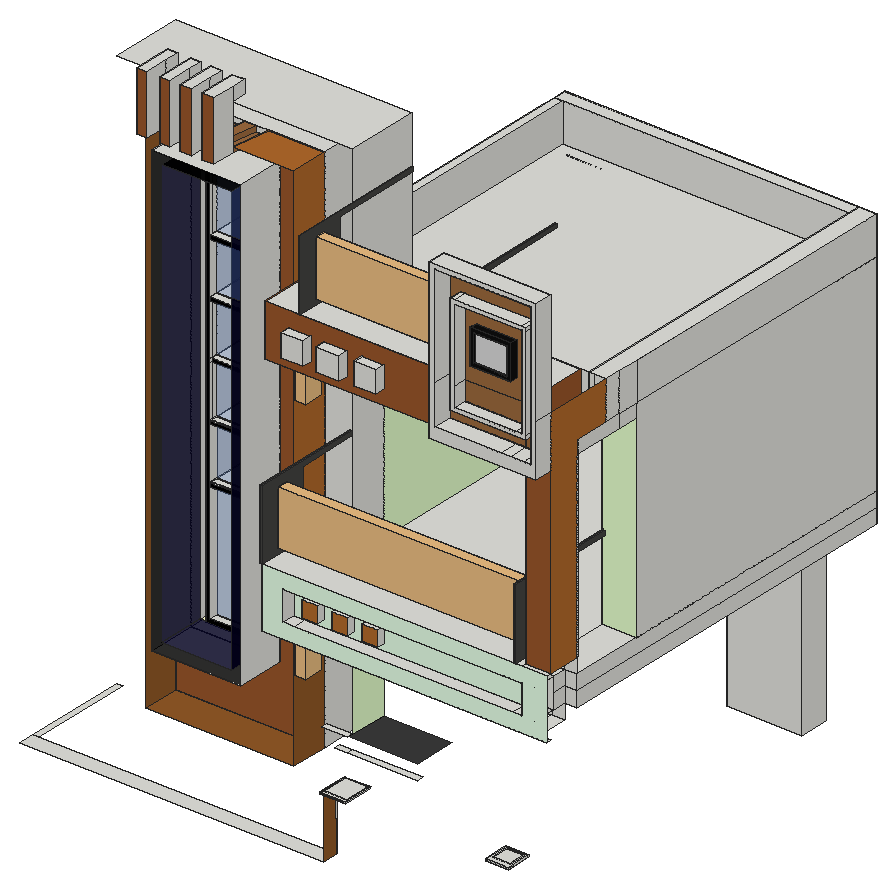
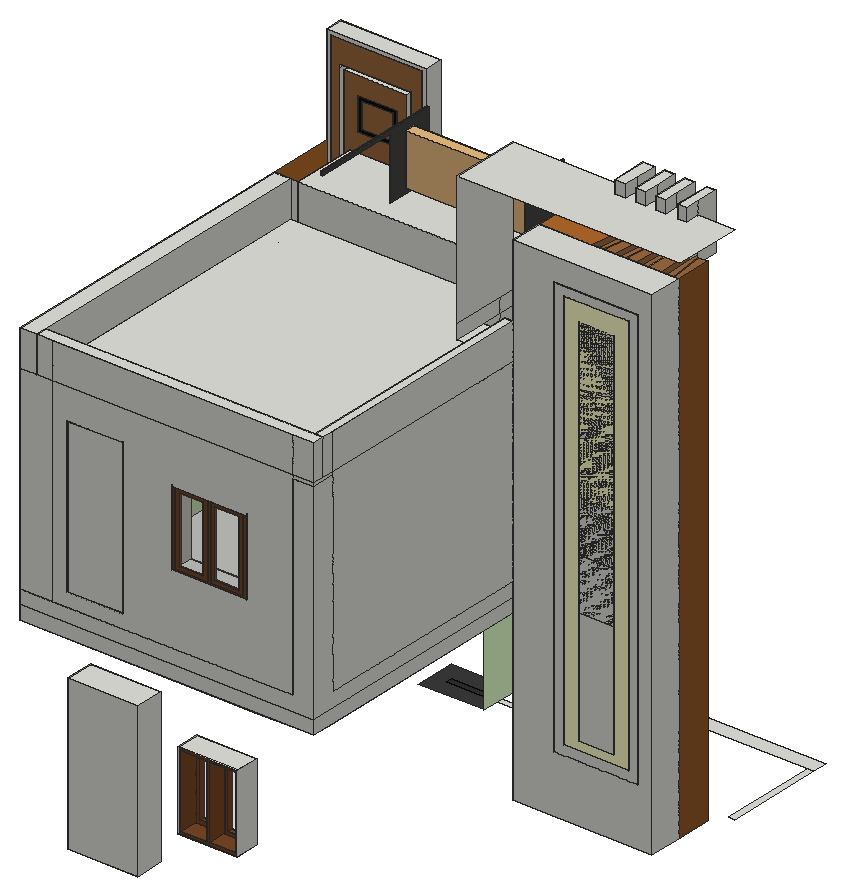
# SketchUp Ruby script. Lengths in inches.
U = 1.inch
M = Sketchup.active_model
def pt(a) = Geom::Point3d.new(a.map { |v| v * U })
def face(e, loops, mat)
  f = e.add_face(loops[0].map { |a| pt(a) })
  loops[1..].each { |l| e.add_face(l.map { |a| pt(a) }).erase! }
  f.material = f.back_material = mat if mat
  f
end
# faces: each face lists its corners as indices into pts; further lists are holes
def faces(e, pts, list, mat = nil) = list.each { |f| face(e, (f[0].is_a?(Array) ? f : [f]).map { |l| l.map { |i| pts[i] } }, mat) }
# xy, xz, yz: faces in a plane at the given z, y or x. An outline is a flat list of corners, or four numbers for a rectangle; further outlines are holes
def ring(l) = l.size == 4 ? [[l[0], l[1]], [l[2], l[1]], [l[2], l[3]], [l[0], l[3]]] : l.each_slice(2).to_a
def flat(e, list, mat, &to3) = list.each { |f| face(e, (f[0].is_a?(Array) ? f : [f]).map { |l| ring(l).map { |u, v| to3.(u, v) } }, mat) }
def xy(e, z, list, mat = nil) = flat(e, list, mat) { |x, y| [x, y, z] }
def xz(e, y, list, mat = nil) = flat(e, list, mat) { |x, z| [x, y, z] }
def yz(e, x, list, mat = nil) = flat(e, list, mat) { |y, z| [x, y, z] }
def lines(e, pts, list) = list.each { |a, b| e.add_line(pt(pts[a]), pt(pts[b])) }
# prism: a flat outline (further loops are holes) pulled along v
def prism(e, loops, v, mat = nil)
  f = face(e, loops, mat); d = Geom::Vector3d.new(v.map { |x| x * U })
  f.pushpull(f.normal.samedirection?(d) ? d.length : -d.length)
end
def box(e, o, s, mat = nil) = prism(e, [[o, [o[0] + s[0], o[1], o[2]], [o[0] + s[0], o[1] + s[1], o[2]], [o[0], o[1] + s[1], o[2]]]], [0, 0, s[2]], mat)
def at(x, y, z, deg = 0) = Geom::Transformation.translation(pt([x, y, z])) * Geom::Transformation.rotation(ORIGIN, Z_AXIS, deg.degrees)
def axes(o, x, y, z) = Geom::Transformation.new([*x, 0, *y, 0, *z, 0, *pt(o).to_a, 1])
def part(name) = M.definitions.add(name)
# library, detail: a bought-in or finely detailed component or shape, given as its bounding box
def library(name, o, s) = part(name).tap { |d| box(d.entities, o, s) }
def detail(e, o, s) = box(e.add_group.entities, o, s)
def put(e, d, t, mat = nil) = e.add_instance(d, t).tap { |i| i.material = mat if mat }
def group(e, t, mat = nil) = e.add_group.tap { |g| g.transformation = t; g.material = mat if mat }.entities
root = M.entities
M.materials.add("MOLDURA PRETA").color = [15, 15, 15]
M.materials.add("[Color E01]").color = [255, 255, 204]
M.materials.add("[Color E03]").color = [229, 255, 230]
M.materials.add("[Color F01]1").color = [229, 255, 204]
M.materials.add("[Color I07]").color = [0, 0, 0]
M.materials["[Color I07]"].alpha = 0.79
M.materials.add("[Color J08]").color = [2, 0, 36]
M.materials["[Color J08]"].alpha = 0.79
M.materials.add("[Color M09]").color = [0, 0, 0]
M.materials.add("[Metal Seamed]2").color = [68, 68, 66]
M.materials.add("[Translucent Glass Blue]").color = [100, 149, 237]
M.materials["[Translucent Glass Blue]"].alpha = 0.28
M.materials.add("[Translucent Glass Gray]").color = [132, 132, 132]
M.materials["[Translucent Glass Gray]"].alpha = 0.25
M.materials.add("[Wood Bamboo]").color = [177, 105, 43]
M.materials.add("[Wood Cherry Original]").color = [152, 86, 42]
M.materials.add("[Wood Floor Parquet]").color = [145, 89, 39]
M.materials.add("[Wood Floor]").color = [155, 105, 61]
M.materials.add("[Wood Veneer 01]").color = [120, 70, 37]
M.materials.add("arvore preta").color = [217, 217, 217]
c1 = part("DOOR12")
g1 = group(c1.entities,at(114.73,28.14,-0.51))
g2 = group(g1,at(0,0,0))
box(g2,[0,0,0],[36,0.5,77.7])
c2 = part("Group\#8")
xy(c2.entities,0,[[0,0,19.69,1.18]],"[Wood Veneer 01]")
xy(c2.entities,2.76,[[2.76,0,16.93,1.18]],"[Wood Veneer 01]")
xy(c2.entities,60.24,[[2.76,0,16.93,1.18]],"[Wood Veneer 01]")
xy(c2.entities,62.99,[[0,0,19.69,1.18]],"[Wood Veneer 01]")
xz(c2.entities,0,[[2.76,2.76,16.93,60.24]],"[Translucent Glass Gray]")
xz(c2.entities,0,[[[0,0,19.69,62.99],[2.76,2.76,16.93,60.24]]],"[Wood Veneer 01]")
xz(c2.entities,1.18,[[[0,0,19.69,62.99],[2.76,2.76,16.93,60.24]]],"[Wood Veneer 01]")
yz(c2.entities,0,[[0,0,1.18,62.99]],"[Wood Veneer 01]")
yz(c2.entities,2.76,[[0,2.76,1.18,60.24]],"[Wood Veneer 01]")
yz(c2.entities,16.93,[[0,2.76,1.18,60.24]],"[Wood Veneer 01]")
yz(c2.entities,19.69,[[0,0,1.18,62.99]],"[Wood Veneer 01]")
c3 = part("pintu 2")
put(c3.entities,c2,at(-19.69,0,1.97))
g3 = group(c3.entities,at(-21.65,0,0))
prism(g3,[[[0,0,66.93],[0,0,0],[45.28,0,0],[45.28,0,66.93]],[[43.31,0,1.97],[23.62,0,1.97],[23.62,0,64.96],[43.31,0,64.96]],[[21.65,0,64.96],[21.65,0,1.97],[1.97,0,1.97],[1.97,0,64.96]]],[0,5.91,0],"[Wood Veneer 01]")
put(c3.entities,c2,at(1.97,0,1.97))
c4 = library("Wall+Light",[81.37,10.74,0],[4.72,6.69,7.875])
c5 = part("Vertical support bracket")
prism(c5.entities,[[[0.39,10.04,41.34],[0.39,0,41.34],[0.39,0,0],[0.39,3.54,0],[0.39,3.54,38.58],[0.39,10.04,38.98]]],[-0.39,0,0],"[Metal Seamed]2")
c6 = part("Link_to_node_rj4\#1")
put(c6.entities,c5,at(2.36,0,0))
c7 = part("Link_to_node_rj8\#1")
put(c7.entities,c5,at(-2.36,0,0),"[Metal Seamed]2")
c8 = library("Horizontal grille bars",[-150.39,-2.17,3.54],[41.02,0.79,32.29])
c9 = part("Agrupar\#1")
prism(c9.entities,[[[14.17,0,12.2],[0,0,12.2],[0,0,0],[14.17,0,0]],[[1.18,0,1.18],[1.18,0,11.02],[12.99,0,11.02],[12.99,0,1.18]]],[0,0.79,0])
c10 = part("Agrupar\#4")
xz(c10.entities,0,[[0,0,11.8125,9.84]],"arvore preta")
c11 = part("Agrupar\#6")
put(c11.entities,c9,at(0,0,0),"MOLDURA PRETA")
put(c11.entities,c10,at(1.18,0.2,1.18))
xy(root,12.68,[[11.58,65.625,71,79.8125]])
xy(root,12.68,[[11.58,50.4375,71,65.625]],"[Wood Floor Parquet]")
xy(root,17.375,[[0,2.125,121.48,8.54],[0,8.54,2.44,50.4375]])
xy(root,26.05,[[103.63,175.125,128.94,185.625]])
xy(root,26.81,[[89.3,47.875,94.55,50.4375],[94.55,47.875,122.48,50.4375]])
xy(root,32.52,[[84.05,47.875,94.55,50.4375]])
xy(root,32.52,[[94.55,47.875,122.48,65.625]],"[Color I07]")
xy(root,37.35,[[17.51,46.0625,53.28,65.625],[17.51,65.625,53.28,79.8125]])
xy(root,41.3,[[21.46,65.625,49.33,79.8125]],"[Color E01]")
xy(root,41.3,[[21.46,46.0625,49.33,65.625]],"[Color J08]")
xy(root,42.0625,[[[187.91,0,197.0625,10.15],[189.03,2.125,196.0625,9.15]]])
xy(root,42.1875,[[120.98,0.77,131.48,2.125],[120.99,2.125,121.48,12.5],[130.61,2.125,131.48,12.75]])
xy(root,42.8125,[[[187.91,0,197.0625,10.15],[189.03,2.125,196.0625,9.15]],[120.98,0.77,131.48,2.125],[120.99,2.125,121.48,12.5],[121.48,2.125,130.61,2.125,130.61,12.75,121.49,12.5,121.49,8.29,121.48,8.54],[130.61,2.125,131.48,12.75],
  [189.03,2.125,196.0625,9.15],[121.49,8.29,121.49,12.5,121.48,12.5,121.48,8.54],[120.99,12.5,121.49,12.5,130.61,12.75,131.48,12.75,131.48,13.3125,130.61,13.3125,121.49,13.0625,120.99,13.0625]])
xy(root,45.21,[[27.72,62.3125,42.78,65.625],[27.72,65.625,42.78,65.6875],[27.72,65.6875,42.78,79.8125]])
xy(root,58.99,[[103.63,175.125,128.94,185.625]])
xy(root,70.2,[[144.35,175.125,174.23,185.625]])
xy(root,78.0625,[[81.61,20.8125,185.87,22.6875],[185.87,20.8125,191,22.6875],[191,20.8125,195.87,22.6875],[185.87,22.6875,191,35.6875],[81.61,35.6875,85.8,50.4375]])
xy(root,84,[[94.55,20.8125,182,26.375],[182,20.8125,185.87,26.375],[94.55,26.375,182,30.1875],[94.55,30.1875,182,35.6875],[182,30.1875,185.87,35.6875],
  [185.87,30.1875,191,35.6875],[94.55,35.6875,182,175.125],[182,35.6875,195.87,65.625],[71,65.625,80,175.4375],[80,65.625,94.55,175.4375],
  [182,65.625,195.87,185.625],[94.55,175.125,182,185.625],[71,175.4375,80,185.625],[80,175.4375,94.55,185.625]])
xy(root,86.45,[[107.64,23.25,114.2,26.375]])
xy(root,86.66,[[95.79,23.25,102.23,26.375]])
xy(root,86.68,[[120,23.25,126.31,26.375]])
xy(root,92.58,[[27.72,62.3125,42.78,63.125],[27.72,63.125,42.78,65.625]])
xy(root,92.99,[[120,23.25,126.31,26.375]])
xy(root,93.02,[[107.64,23.25,114.2,26.375]])
xy(root,93.1,[[95.79,23.25,102.23,26.375]])
xy(root,94.05,[[26,62.3125,26.22,65.625],[27.72,62.3125,42.78,63.125],[27.72,63.125,42.78,65.625]])
xy(root,94.08,[[27.72,65.625,42.78,65.6875],[27.72,65.6875,42.78,79.8125]])
xy(root,96,[[90.17,20.8125,94.55,26.375],[94.55,20.8125,182,26.375],[182,20.8125,185.87,26.375],[90.17,26.375,94.55,30.1875],[94.55,26.375,182,30.1875],
  [90.17,30.1875,94.55,35.6875],[94.55,30.1875,182,35.6875],[182,30.1875,185.87,35.6875],[185.87,30.1875,191,35.6875],[94.55,35.6875,182,175.5625],
  [182,35.6875,195.87,65.625],[71,65.625,80,175.5625],[80,65.625,94.55,175.5625],[182,65.625,195.87,185.625],[80,175.5625,182,176.625],
  [80,176.625,182,185.625]])
xy(root,101.82,[[152.16,175.5625,175.85,185.625]])
xy(root,102,[[81.61,20.8125,185.87,35.6875],[185.87,20.8125,195.87,22.6875],[185.87,22.6875,195.87,35.6875],[81.61,35.6875,85.8,50.4375]])
xy(root,114.9,[[27.72,62.3125,42.78,63.125],[27.72,63.125,42.78,65.625]])
xy(root,116.27,[[27.72,62.3125,42.78,63.125],[27.72,63.125,42.78,65.625],[27.72,65.625,42.78,79.8125]])
xy(root,116.33,[[26.22,62.3125,26.28,65.625],[44.22,62.3125,44.28,65.625],[26.28,63.125,27.72,65.625]])
xy(root,125.65,[[99.56,175.5625,131.49,185.625]])
xy(root,136.99,[[26.25,62.3125,26.28,63.125],[44.22,62.3125,44.25,65.625],[26.25,63.125,26.28,65.625]])
xy(root,137.02,[[27.72,63.125,42.78,65.625]])
xy(root,138.43,[[27.72,63.125,42.78,65.625]])
xy(root,138.46,[[27.72,65.625,42.78,79.8125]])
xy(root,157.59,[[99.56,175.5625,131.49,185.625]])
xy(root,159.2,[[26.27,63.125,27.72,65.625],[42.78,63.125,44.23,65.625]])
xy(root,159.27,[[27.72,62.3125,42.78,65.625]])
xy(root,160.65,[[27.72,62.3125,42.78,65.625],[27.72,65.625,42.78,79.8125]])
xy(root,160.67,[[26.25,62.3125,26.27,63.125],[44.23,62.3125,44.25,65.625],[26.25,63.125,26.27,65.625],[26.27,63.125,27.72,65.625],[42.78,63.125,44.23,65.625]])
xy(root,167.13,[[152.16,175.5625,175.85,185.625]])
xy(root,174.6875,[[153.06,15.1875,182,22.6875],[182,15.1875,185.87,22.6875],[185.87,15.1875,191,22.6875],[191,15.1875,195.87,22.6875],[182,56.9375,195.87,65.625]])
xy(root,174.6875,[[81.61,22.6875,81.61,50.4375,94.55,50.4375,94.55,56.9375,182,56.9375,182,22.6875],[94.55,56.9375,182,175.5625]],"[Color E03]")
xy(root,178.6875,[[71,175.5625,80,185.625]])
xy(root,179.5625,[[155.37,15.1875,182,22.6875],[182,15.1875,185.87,22.6875],[185.87,15.1875,191,22.6875],[191,15.1875,193.99,22.6875]])
xy(root,179.92,[[105.19,18.6875,114.44,22.6875]])
xy(root,180,[[185.87,35.6875,191,36.0625],[191,35.6875,195.87,36.0625],[185.87,36.0625,191,50.4375],[191,36.0625,195.87,50.4375],[94.55,50.4375,188.93,50.4375,188.93,180.59,74.48,180.59,74.48,79.8125,94.55,79.8125],
  [188.93,50.4375,195.87,185.625],[71,65.625,94.55,79.8125],[71,79.8125,74.48,180.59],[71,180.59,188.93,185.625]])
xy(root,180.16,[[90.875,18.6875,99.875,22.6875]])
xy(root,180.49,[[120.34,18.6875,129.03,22.6875]])
xy(root,181.38,[[27.72,62.3125,42.78,65.625],[42.78,63.125,44.23,65.625]])
xy(root,182.83,[[27.72,62.3125,42.78,65.625],[26.27,63.125,27.72,65.625],[42.78,63.125,44.23,65.625],[27.72,65.625,42.78,79.8125]])
xy(root,186.11,[[159.87,17.4375,161.49,22.6875],[161.49,17.4375,185.87,22.6875],[185.87,17.4375,188.56,22.6875],[188.56,17.4375,190.18,22.6875]])
xy(root,187.55,[[161.49,17.4375,185.87,22.6875],[185.87,17.4375,188.56,22.6875]])
xy(root,189.16,[[90.875,18.6875,99.875,22.6875]])
xy(root,189.17,[[105.19,18.6875,114.44,22.6875]])
xy(root,189.18,[[120.34,18.6875,129.03,22.6875]])
xy(root,195.375,[[81.61,22.6875,185.87,50.4375],[188.93,50.4375,195.87,185.625],[71,79.8125,74.48,180.59],[71,180.59,188.93,185.625]])
xy(root,205.02,[[27.72,62.3125,42.78,63.125],[27.72,63.125,42.78,65.625],[27.72,65.625,42.78,79.8125]])
xy(root,206.47,[[26.27,62.3125,44.23,63.125],[26.27,63.125,44.23,65.625]])
xy(root,212.8,[[21.46,65.625,49.33,79.8125]])
xy(root,212.8,[[21.46,46.0625,49.33,65.625]],"[Color I07]")
xy(root,216.74,[[17.51,46.0625,53.28,65.625],[17.51,65.625,53.28,79.8125]])
xy(root,223.99,[[15.47,41.0625,15.47,50.4375,13.73,65.625,18.71,65.625,19.49,50.4375,19.49,41.0625],[24.63,41.0625,24.63,65.625,29.625,65.625,28.7,50.4375,28.7,41.0625],[32.79,41.0625,32.79,50.4375,34.02,65.625,39.01,65.625,37.31,50.4375,37.31,41.0625],[41.38,41.0625,41.38,50.4375,43.62,65.625,48.59,65.625,46.35,50.4375,46.35,41.0625]],"[Wood Floor]")
xy(root,224.86,[[161.49,17.4375,188.56,22.6875]])
xy(root,226.18,[[11.58,65.625,71,79.8125]])
xy(root,226.18,[[46.35,50.4375,48.59,65.625,71,65.625,71,50.4375]],"[Wood Bamboo]")
xy(root,226.18,[[11.58,50.4375,11.58,65.625,13.73,65.625,15.47,50.4375],[19.49,50.4375,18.71,65.625,24.63,65.625,24.63,50.4375],[28.7,50.4375,29.625,65.625,34.02,65.625,32.79,50.4375],[37.31,50.4375,39.01,65.625,43.62,65.625,41.38,50.4375]],"[Wood Floor]")
xy(root,226.35,[[159.87,17.4375,161.49,22.6875],[161.49,17.4375,188.56,22.6875],[188.56,17.4375,190.18,22.6875]])
xy(root,236.25,[[155.37,15.1875,193.99,22.6875]])
xy(root,237.8125,[[153.06,15.1875,195.87,22.6875]])
xy(root,242.375,[[0,50.4375,15.47,50.4375,15.47,56.4375,19.49,56.4375,19.49,50.4375,24.63,50.4375,24.63,56.4375,28.7,56.4375,28.7,50.4375,32.79,50.4375,32.79,56.4375,37.31,56.4375,37.31,50.4375,41.38,50.4375,41.38,56.4375,46.35,56.4375,46.35,50.4375,94.55,50.4375,94.55,79.8125,0,79.8125]])
xy(root,247.75,[[15.47,41.0625,19.49,56.4375],[24.63,41.0625,28.7,56.4375],[32.79,41.0625,37.31,56.4375],[41.38,41.0625,46.35,56.4375]])
xz(root,0,[[187.91,42.0625,188.41,42.8125],[188.41,42.0625,195.4375,42.8125],[195.4375,42.0625,197.0625,42.8125]])
xz(root,0.77,[[120.98,42.1875,121.48,42.8125],[121.48,42.1875,130.61,42.8125],[130.61,42.1875,131.48,42.8125]])
xz(root,2.125,[[189.03,42.0625,196.0625,42.8125],[120.98,42.1875,120.99,42.8125],[120.99,42.1875,121.48,42.8125],[121.48,42.1875,130.61,42.8125],[130.61,42.1875,131.48,42.8125]])
xz(root,9.15,[[189.03,42.0625,196.0625,42.8125]])
xz(root,10.15,[[187.91,42.0625,189.03,42.8125],[189.03,42.0625,196.0625,42.8125],[196.0625,42.0625,197.0625,42.8125]])
xz(root,12.5,[[120.99,42.1875,121.48,42.8125]])
xz(root,12.75,[[130.61,42.1875,131.48,42.8125]])
xz(root,15.1875,[[[153.06,174.6875,195.87,237.8125],[155.37,179.5625,193.99,236.25]]])
xz(root,17.4375,[[[159.87,186.11,190.18,226.35],[161.49,187.55,188.56,224.86]]])
xz(root,18.6875,[[105.19,179.92,114.44,189.17],[90.875,180.16,99.875,189.16],[120.34,180.49,129.03,189.18]])
xz(root,20.8125,[[[81.61,78.0625,195.87,102],[94.55,84,90.17,84.03,90.17,96,185.87,96,185.87,84]]],"[Color E03]")
xz(root,22.6875,[[153.06,174.6875,153.06,195.375,155.37,195.375,155.37,179.5625,185.87,179.5625,185.87,174.6875],[185.87,174.6875,185.87,179.5625,193.99,179.5625,193.99,236.25,155.37,236.25,155.37,195.375,153.06,195.375,153.06,237.8125,195.87,237.8125,195.87,174.6875],[159.87,186.11,159.87,195.375,161.49,195.375,161.49,187.55,185.87,187.55,185.87,186.11]])
xz(root,22.6875,[[185.87,102,195.87,174.6875],[[81.61,174.6875,153.06,195.375],[105.19,179.92,114.44,189.17],[90.875,180.16,99.875,189.16],[120.34,180.49,129.03,189.18]]],"[Wood Cherry Original]")
xz(root,22.6875,[[155.37,179.5625,185.87,179.5625,185.87,186.11,159.87,186.11,159.87,195.375,155.37,195.375],[185.87,179.5625,193.99,179.5625,193.99,236.25,155.37,236.25,155.37,195.375,159.87,195.375,159.87,226.35,190.18,226.35,190.18,186.11,185.87,186.11],[161.49,187.55,185.87,195.375],[185.87,187.55,188.56,187.55,188.56,224.86,161.49,224.86,161.49,195.375,185.87,195.375]],"[Wood Floor]")
xz(root,23.25,[[107.64,86.45,114.2,93.02],[95.79,86.66,102.23,93.1],[120,86.68,126.31,92.99]],"[Wood Bamboo]")
xz(root,26.375,[[[94.55,84,185.87,84,185.87,96,90.17,96,90.17,84.03],[107.64,86.45,114.2,93.02],[95.79,86.66,102.23,93.1],[120,86.68,126.31,92.99]]],"[Color E03]")
xz(root,30.1875,[[94.55,84,191,84,191,96,90.17,96,90.17,84.03]])
xz(root,35.6875,[[85.8,78.0625,85.8,102,185.87,102,185.87,96,90.17,96,90.17,84.03,94.55,84,185.87,84,185.87,78.0625],[185.87,78.0625,191,84],[94.55,84,90.17,84.03,90.17,96,185.87,96,185.87,84],[185.87,84,191,96],[191,84,195.87,90],
  [191,90,195.87,96],[191,96,195.87,102],[185.87,102,191,174.6875],[191,102,195.87,174.6875],[185.87,174.6875,191,180],
  [191,174.6875,195.87,180]])
xz(root,41.0625,[[15.47,223.99,19.49,247.75],[24.63,223.99,28.7,247.75],[32.79,223.99,37.31,247.75],[41.38,223.99,46.35,247.75]],"[Wood Cherry Original]")
xz(root,46.0625,[[[17.51,37.35,53.28,216.74],[21.46,41.3,49.33,212.8]]],"[Color I07]")
xz(root,50.4375,[[81.61,174.6875,94.55,180],[81.61,180,94.55,195.375],[94.55,180,185.87,195.375],[185.87,180,188.93,195.375],[188.93,180,191,195.375],
  [191,180,195.87,195.375]])
xz(root,50.4375,[[19.49,226.18,24.63,242.375],[28.7,226.18,32.79,242.375],[37.31,226.18,41.38,242.375]],"[Color I07]")
xz(root,56.4375,[[15.47,242.375,19.49,247.75],[24.63,242.375,28.7,247.75],[32.79,242.375,37.31,247.75],[41.38,242.375,46.35,247.75]])
xz(root,62.3125,[[[26,43.49,44.35,43.53,44.35,94.09,44.28,94.05,44.28,116.33,44.22,116.33,44.22,136.99,44.25,136.99,44.25,160.67,44.23,160.67,44.23,206.47,26.27,206.47,26.27,160.67,26.25,160.67,26.25,136.99,26.28,136.99,26.28,116.33,26.22,116.33,26.22,94.05,26,94.05],[27.72,45.21,42.78,181.38],[27.72,182.83,42.78,205.02]],[27.72,92.58,42.78,94.05],[27.72,114.9,42.78,116.27],[27.72,159.27,42.78,160.65]],"[Color M09]")
xz(root,63.125,[[27.72,92.58,42.78,94.05],[27.72,114.9,42.78,116.27],[26.28,116.33,26.28,136.99,26.25,136.99,26.25,160.67,26.27,160.67,26.27,159.2,27.72,159.2,27.72,116.33],[26.27,159.2,27.72,160.67],[42.78,159.2,44.23,160.67],
  [42.78,181.38,44.23,182.83],[26.27,182.83,26.27,206.47,44.23,206.47,44.23,182.83,42.78,182.83,42.78,205.02,27.72,205.02,27.72,182.83]])
xz(root,63.125,[[27.72,137.02,42.78,138.43]],"[Color M09]")
xz(root,65.625,[[26,43.49,26,94.05,26.22,94.05,26.22,92.58,27.72,92.58,27.72,45.21,42.78,45.21,42.78,92.58,44.28,92.58,44.28,94.05,44.35,94.09,44.35,43.53],[71,90,94.55,96],[42.78,92.58,44.28,94.05],[26.22,94.05,27.72,116.33],[27.72,94.05,42.78,94.08],
  [42.78,94.05,42.78,136.99,44.22,136.99,44.22,116.33,44.28,116.33,44.28,94.05],[71,96,94.55,180],[27.72,114.83,42.78,114.9],[27.72,114.9,42.78,116.27],[27.72,116.27,42.78,116.33],
  [26.28,116.33,27.72,136.99],[26.25,136.99,26.25,160.67,26.27,160.67,26.27,159.2,27.72,159.2,27.72,138.43,26.28,138.43,26.28,136.99],[26.28,136.99,27.72,138.43],[27.72,136.99,42.78,137.02],[42.78,136.99,44.22,138.43],
  [44.22,136.99,44.22,138.43,42.78,138.43,42.78,159.2,44.23,159.2,44.23,160.67,44.25,160.67,44.25,136.99],[27.72,137.02,42.78,138.43],[27.72,138.43,42.78,138.46],[27.72,159.2,42.78,159.27],[27.72,159.27,42.78,160.65],
  [27.72,160.65,42.78,160.67],[26.27,160.67,26.27,181.38,27.72,181.38,27.72,182.83,42.78,182.83,42.78,181.38,44.23,181.38,44.23,160.67,42.78,160.67,42.78,181.38,27.72,181.38,27.72,160.67],[27.72,181.38,42.78,182.83],[42.78,181.38,44.23,182.83],[26.27,182.83,26.27,206.47,44.23,206.47,44.23,182.83,42.78,182.83,42.78,205.02,27.72,205.02,27.72,182.83],
  [13.73,223.99,18.71,226.18],[24.63,223.99,29.625,226.18],[34.02,223.99,39.01,226.18],[43.62,223.99,48.59,226.18]])
xz(root,65.625,[[182,96,195.87,174.6875]],"[Color F01]1")
xz(root,65.625,[[27.72,45.21,42.78,92.58],[27.72,94.08,42.78,114.83],[27.72,116.33,42.78,136.99],[27.72,138.46,42.78,159.2],[27.72,160.67,42.78,181.38],
  [27.72,182.83,42.78,205.02]],"[Translucent Glass Blue]")
xz(root,65.625,[[[11.58,12.68,71,12.68,71,226.18,48.59,226.18,48.59,223.99,43.62,223.99,43.62,226.18,39.01,226.18,39.01,223.99,34.02,223.99,34.02,226.18,29.625,226.18,29.625,223.99,24.63,223.99,24.63,226.18,18.71,226.18,18.71,223.99,13.73,223.99,13.73,226.18,11.58,226.18],[17.51,37.35,53.28,216.74]]],"[Wood Cherry Original]")
xz(root,65.6875,[[27.72,45.21,42.78,94.08]])
xz(root,79.8125,[[[11.58,12.68,71,226.18],[17.51,37.35,53.28,216.74]],[[17.51,37.35,53.28,216.74],[21.46,41.3,49.33,212.8]],[27.72,45.21,42.78,94.08],[27.72,94.08,42.78,116.27],[27.72,116.27,42.78,138.46],
  [27.72,138.46,42.78,160.65],[27.72,160.65,42.78,182.83],[71,180,74.48,195.375],[27.72,182.83,42.78,205.02]])
xz(root,79.8125,[[[21.46,41.3,49.33,212.8],[27.72,45.21,42.78,94.08]]],"[Color E01]")
xz(root,175.5625,[[71,96,80,178.6875],[80,96,94.55,180]])
xz(root,175.5625,[[[94.55,96,182,174.6875],[152.16,101.82,175.85,167.13],[99.56,125.65,131.49,157.59]]],"[Color F01]1")
xz(root,180.59,[[71,180,74.48,195.375],[74.48,180,188.93,195.375]])
xz(root,185.625,[[71,84,195.87,90],[71,90,71,178.6875,80,178.6875,80,96,195.87,96,195.87,90],[[80,96,182,180],[152.16,101.82,175.85,167.13],[99.56,125.65,131.49,157.59]],[182,96,195.87,180],[71,178.6875,80,180],
  [71,180,80,195.375],[80,180,182,195.375],[182,180,188.93,195.375],[188.93,180,195.87,195.375]])
yz(root,11.58,[[65.625,12.68,79.8125,226.18]])
yz(root,11.58,[[50.4375,12.68,65.625,226.18]],"[Wood Floor Parquet]")
yz(root,15.47,[[41.0625,223.99,50.4375,247.75],[50.4375,242.375,56.4375,247.75]])
yz(root,17.51,[[46.0625,37.35,65.625,216.74],[65.625,37.35,79.8125,216.74]])
yz(root,19.49,[[41.0625,223.99,50.4375,247.75],[50.4375,242.375,56.4375,247.75]])
yz(root,21.46,[[65.625,41.3,79.8125,212.8]])
yz(root,21.46,[[46.0625,41.3,65.625,212.8]],"[Color J08]")
yz(root,24.63,[[41.0625,223.99,50.4375,247.75],[50.4375,223.99,65.625,226.18],[50.4375,242.375,56.4375,247.75]])
yz(root,26,[[62.3125,43.49,65.625,94.05]])
yz(root,26.22,[[62.3125,94.05,65.625,116.33]])
yz(root,26.25,[[62.3125,136.99,63.125,160.67],[63.125,136.99,65.625,160.67]])
yz(root,26.27,[[62.3125,159.2,63.125,160.67],[63.125,159.2,65.625,160.67],[62.3125,160.67,65.625,181.38],[62.3125,181.38,65.625,182.83],[62.3125,182.83,63.125,206.47],
  [63.125,182.83,65.625,206.47]])
yz(root,26.28,[[62.3125,116.33,63.125,136.99],[63.125,116.33,65.625,136.99],[63.125,136.99,65.625,138.43]])
yz(root,27.72,[[62.3125,45.21,65.625,92.33],[65.625,45.21,65.6875,45.21,65.6875,94.08,65.625,94.08,65.625,94.05,63.125,94.05,63.125,92.58,65.625,92.58],[65.6875,45.21,79.8125,94.08],[62.3125,92.33,65.625,92.58],[62.3125,92.58,63.125,94.05],
  [62.3125,94.05,65.625,94.08],[62.3125,94.08,65.625,114.83],[65.625,94.08,79.8125,116.27],[62.3125,114.83,65.625,114.9],[62.3125,114.9,63.125,116.27],
  [63.125,114.9,65.625,116.27],[62.3125,116.27,65.625,116.33],[65.625,116.27,79.8125,138.46],[62.3125,116.33,63.125,136.99],[63.125,116.33,65.625,136.99],
  [62.3125,136.99,63.125,137.02],[63.125,136.99,65.625,137.02],[62.3125,137.02,63.125,138.43],[63.125,137.02,65.625,138.43],[62.3125,138.43,63.125,138.46],
  [63.125,138.43,65.625,138.46],[62.3125,138.46,63.125,159.2],[63.125,138.46,65.625,159.2],[65.625,138.46,79.8125,160.65],[62.3125,159.2,63.125,159.27],
  [63.125,159.2,65.625,159.27],[62.3125,159.27,63.125,160.65],[63.125,159.27,65.625,160.65],[62.3125,160.65,63.125,160.67],[63.125,160.65,65.625,160.67],
  [65.625,160.65,79.8125,182.83],[62.3125,160.67,65.625,181.38],[62.3125,181.38,65.625,182.83],[62.3125,182.83,63.125,205.02],[63.125,182.83,65.625,205.02],
  [65.625,182.83,79.8125,205.02]])
yz(root,28.7,[[41.0625,223.99,50.4375,247.75],[50.4375,242.375,56.4375,247.75]])
yz(root,32.79,[[41.0625,223.99,50.4375,247.75],[50.4375,242.375,56.4375,247.75]])
yz(root,37.31,[[41.0625,223.99,50.4375,247.75],[50.4375,242.375,56.4375,247.75]])
yz(root,41.38,[[41.0625,223.99,50.4375,247.75],[50.4375,242.375,56.4375,247.75]])
yz(root,42.78,[[62.3125,45.21,65.625,92.33],[65.625,45.21,65.6875,94.08],[65.6875,45.21,79.8125,94.08],[62.3125,92.33,65.625,92.58],[62.3125,92.58,63.125,94.05],
  [63.125,92.58,65.625,94.05],[62.3125,94.05,65.625,94.08],[62.3125,94.08,65.625,114.83],[65.625,94.08,79.8125,116.27],[62.3125,114.83,65.625,114.9],
  [62.3125,114.9,63.125,116.27],[63.125,114.9,65.625,116.27],[62.3125,116.27,65.625,116.33],[65.625,116.27,79.8125,138.46],[62.3125,116.33,65.625,136.99],
  [62.3125,136.99,65.625,137.02],[62.3125,137.02,63.125,138.43],[63.125,137.02,65.625,138.43],[62.3125,138.43,65.625,138.46],[62.3125,138.46,65.625,159.2],
  [65.625,138.46,79.8125,160.65],[62.3125,159.2,63.125,159.27],[63.125,159.2,65.625,159.27],[62.3125,159.27,63.125,160.65],[63.125,159.27,65.625,160.65],
  [62.3125,160.65,63.125,160.67],[63.125,160.65,65.625,160.67],[65.625,160.65,79.8125,182.83],[62.3125,160.67,65.625,181.38],[62.3125,181.38,63.125,182.83],
  [63.125,181.38,65.625,182.83],[62.3125,182.83,63.125,205.02],[63.125,182.83,65.625,205.02],[65.625,182.83,79.8125,205.02]])
yz(root,44.22,[[62.3125,116.33,65.625,136.99],[63.125,136.99,65.625,138.43]])
yz(root,44.23,[[62.3125,159.2,63.125,160.67],[63.125,159.2,65.625,160.67],[62.3125,160.67,65.625,181.38],[62.3125,181.38,63.125,182.83],[63.125,181.38,65.625,182.83],
  [62.3125,182.83,63.125,206.47],[63.125,182.83,65.625,206.47]])
yz(root,44.25,[[62.3125,136.99,65.625,160.67]])
yz(root,44.28,[[62.3125,92.58,65.625,94.05],[62.3125,94.05,65.625,116.33]])
yz(root,44.35,[[62.3125,43.53,65.625,94.09]])
yz(root,46.35,[[41.0625,223.99,50.4375,247.75],[50.4375,242.375,56.4375,247.75]])
yz(root,49.33,[[65.625,41.3,79.8125,212.8]])
yz(root,49.33,[[46.0625,41.3,65.625,212.8]],"[Color J08]")
yz(root,53.28,[[46.0625,37.35,65.625,216.74],[65.625,37.35,79.8125,216.74]])
yz(root,71,[[65.625,12.68,79.8125,84],[65.625,84,79.8125,90],[79.8125,84,185.625,90],[65.625,90,79.8125,96],[79.8125,90,79.8125,96,175.5625,96,175.5625,178.6875,185.625,178.6875,185.625,90],
  [65.625,96,79.8125,180],[79.8125,96,175.5625,180],[175.5625,178.6875,185.625,180],[65.625,180,79.8125,226.18],[79.8125,180,175.5625,195.375],
  [175.5625,180,180.59,195.375],[180.59,180,185.625,195.375]])
yz(root,71,[[50.4375,96,65.625,180],[50.4375,180,65.625,226.18]],"[Wood Bamboo]")
yz(root,71,[[50.4375,12.68,65.625,84]],"[Wood Floor Parquet]")
yz(root,71,[[50.4375,84,65.625,90],[50.4375,90,65.625,96]],"[Wood Floor]")
yz(root,74.48,[[79.8125,180,180.59,195.375]])
yz(root,80,[[175.5625,96,176.625,178.6875],[176.625,96,185.625,178.6875]])
yz(root,81.61,[[20.8125,78.0625,35.6875,84.0625],[35.6875,78.0625,35.6875,84.0625,20.8125,84.0625,20.8125,96,35.6875,96,35.6875,102,50.4375,102,50.4375,78.0625],[20.8125,96,35.6875,102]])
yz(root,81.61,[[22.6875,174.6875,50.4375,195.375]],"[Wood Cherry Original]")
yz(root,85.8,[[35.6875,78.0625,50.4375,84.0625],[35.6875,96,50.4375,102]])
yz(root,90.17,[[20.8125,84.03,26.375,96],[26.375,84.03,30.1875,96],[30.1875,84.03,35.6875,96]])
yz(root,90.875,[[18.6875,180.16,22.6875,189.16]])
yz(root,94.55,[[50.4375,96,65.625,174.6875],[50.4375,174.6875,56.9375,180],[56.9375,174.6875,65.625,180],[50.4375,180,56.9375,186],[56.9375,180,79.8125,186],
  [50.4375,186,79.8125,242.375]])
yz(root,94.55,[[50.4375,32.52,65.625,84],[65.625,96,175.5625,174.6875]],"[Color F01]1")
yz(root,95.79,[[23.25,86.66,26.375,93.1]])
yz(root,99.56,[[175.5625,125.65,185.625,157.59]])
yz(root,99.875,[[18.6875,180.16,22.6875,189.16]])
yz(root,102.23,[[23.25,86.66,26.375,93.1]])
yz(root,103.63,[[175.125,26.05,185.625,58.99]])
yz(root,105.19,[[18.6875,179.92,22.6875,189.17]])
yz(root,107.64,[[23.25,86.45,26.375,93.02]])
yz(root,114.2,[[23.25,86.45,26.375,93.02]])
yz(root,114.44,[[18.6875,179.92,22.6875,189.17]])
yz(root,120,[[23.25,86.68,26.375,92.99]])
yz(root,120.34,[[18.6875,180.49,22.6875,189.18]])
yz(root,120.98,[[0.77,42.1875,2.125,42.8125]])
yz(root,120.99,[[2.125,42.1875,8.29,42.8125],[8.29,42.1875,12.5,42.8125]])
yz(root,121.48,[[2.125,42.1875,8.54,42.8125],[8.54,42.1875,12.5,42.8125]])
yz(root,121.48,[[2.125,17.375,8.54,42.1875]],"[Wood Floor Parquet]")
yz(root,126.31,[[23.25,86.68,26.375,92.99]])
yz(root,128.94,[[175.125,26.05,185.625,58.99]])
yz(root,129.03,[[18.6875,180.49,22.6875,189.18]])
yz(root,130.61,[[2.125,42.1875,12.75,42.8125]])
yz(root,131.48,[[0.77,42.1875,2.125,42.8125],[2.125,42.1875,12.75,42.8125]])
yz(root,131.49,[[175.5625,125.65,185.625,157.59]])
yz(root,152.16,[[175.5625,101.82,185.625,167.13]])
yz(root,153.06,[[15.1875,174.6875,22.6875,195.375],[15.1875,195.375,22.6875,237.8125]])
yz(root,155.37,[[15.1875,179.5625,22.6875,195.375],[15.1875,195.375,22.6875,236.25]])
yz(root,159.87,[[17.4375,186.11,22.6875,224.86],[17.4375,224.86,22.6875,226.35]])
yz(root,161.49,[[17.4375,187.55,22.6875,195.375],[17.4375,195.375,22.6875,224.86]])
yz(root,175.85,[[175.5625,101.82,185.625,167.13]])
yz(root,182,[[65.625,96,175.5625,174.6875]],"[Color F01]1")
yz(root,185.87,[[20.8125,84,26.375,96],[26.375,84,35.6875,96]])
yz(root,185.87,[[22.6875,102,22.6875,195.375,50.4375,195.375,50.4375,180,35.6875,180,35.6875,102]],"[Wood Cherry Original]")
yz(root,187.91,[[0,42.0625,2.125,42.8125],[2.125,42.0625,9.15,42.8125],[9.15,42.0625,10.15,42.8125]])
yz(root,188.56,[[17.4375,187.55,22.6875,224.86]])
yz(root,188.93,[[50.4375,180,180.59,195.375],[180.59,180,185.625,195.375]])
yz(root,189.03,[[2.125,42.0625,9.15,42.8125]])
yz(root,190.18,[[17.4375,186.11,22.6875,187.55],[17.4375,187.55,22.6875,224.86],[17.4375,224.86,22.6875,226.35]])
yz(root,191,[[30.1875,84,35.6875,90],[30.1875,90,35.6875,96]])
yz(root,193.99,[[15.1875,179.5625,22.6875,195.375],[15.1875,195.375,22.6875,236.25]])
yz(root,195.87,[[35.6875,84,185.625,90],[35.6875,90,185.625,96],[65.625,96,185.625,180],[35.6875,102,36.0625,174.6875],[15.1875,174.6875,22.6875,195.375],
  [35.6875,174.6875,36.0625,180],[36.0625,174.6875,56.9375,180],[56.9375,174.6875,65.625,180],[50.4375,180,56.9375,195.375],[56.9375,180,65.625,195.375],
  [65.625,180,185.625,195.375],[15.1875,195.375,22.6875,237.8125]])
yz(root,195.87,[[22.6875,102,35.6875,102,35.6875,180,50.4375,180,50.4375,195.375,22.6875,195.375]],"[Wood Bamboo]")
yz(root,196.0625,[[2.125,42.0625,9.15,42.8125]])
yz(root,197.0625,[[0,42.0625,2.125,42.8125],[2.125,42.0625,9.15,42.8125],[9.15,42.0625,10.15,42.8125]])
p = [[121.49,8.29,42.8125],[121.48,8.42,17.375],[121.48,8.54,17.375],[121.48,8.54,42.1875],[121.48,8.54,42.8125],[26,65.625,43.49],
  [44.35,65.625,43.53],[44.35,62.3125,43.53],[26,62.3125,43.49],[90.17,26.375,84.03],[90.17,20.8125,84.03],[94.55,20.8125,84],
  [94.55,26.375,84],[94.55,30.1875,84],[90.17,30.1875,84.03],[94.55,35.6875,84],[90.17,35.6875,84.03],[44.35,65.625,94.09],
  [44.28,65.625,94.05],[44.28,62.3125,94.05],[44.35,62.3125,94.09],[15.47,50.4375,226.18],[13.73,65.625,226.18],[13.73,65.625,223.99],
  [15.47,50.4375,223.99],[18.71,65.625,226.18],[19.49,50.4375,226.18],[19.49,50.4375,223.99],[18.71,65.625,223.99],[29.625,65.625,226.18],
  [28.7,50.4375,226.18],[28.7,50.4375,223.99],[29.625,65.625,223.99],[32.79,50.4375,226.18],[34.02,65.625,226.18],[34.02,65.625,223.99],
  [32.79,50.4375,223.99],[39.01,65.625,226.18],[37.31,50.4375,226.18],[37.31,50.4375,223.99],[39.01,65.625,223.99],[41.38,50.4375,226.18],
  [43.62,65.625,226.18],[43.62,65.625,223.99],[41.38,50.4375,223.99],[48.59,65.625,226.18],[46.35,50.4375,226.18],[46.35,50.4375,223.99],
  [48.59,65.625,223.99],[80,176.625,178.6875],[80,176.625,180],[182,65.625,180],[182,65.625,174.6875],[191,30.1875,84],
  [191,20.8125,84],[191,30.1875,96],[191,20.8125,96],[94.55,65.625,90],[94.55,50.4375,90],[195.87,36.0625,102],
  [191,35.6875,102],[191,35.6875,174.6875],[191,22.6875,174.6875],[120.98,2.125,42.8125],[120.98,8.54,42.8125],[182,175.5625,174.6875],
  [182,175.5625,180],[182,176.625,96],[182,176.625,180],[26.28,65.625,116.33],[26.28,65.625,114.83],[26.22,65.625,92.58],
  [26.22,63.125,92.58]]
faces(root,p,[[0,1,2,3,4],[5,6,7,8],[9,10,11,12],[12,13,14,9],[15,16,14,13],[17,18,19,20]])
faces(root,p,[[21,22,23,24],[25,26,27,28],[29,30,31,32],[33,34,35,36],[37,38,39,40],[41,42,43,44],[45,46,47,48]],"[Wood Floor]")
lines(root,p,[[49,50],[51,52],[53,54],[55,56],[57,58],[59,60],[61,62],[63,64],[65,66],[67,68],[69,70],[71,72]])
put(root,c1,axes([49.14,-511.875,5.58],[0.82986,0,0],[0,24.41523,0],[0,0,0.83722]))
put(root,c3,axes([115.74,175.125,26.05],[0.55908,0,0],[0,1.6895,0],[0,0,0.49212]))
put(root,c4,axes([159.31,30.4,50.82],[-0.95295,0,0],[0,1.15504,0],[0,0,1.83205]))
put(root,c1,axes([76.67,-374.04,102.25],[0.65799,0,0],[0,19.53219,0],[0,0,0.83722]))
put(root,c6,axes([189.15,20.8125,102],[-2.4464,0,0],[0,5.61804,0],[0,0,0.68]))
put(root,c7,axes([76.26,20.8125,102],[-2.4464,0,0],[0,5.61804,0],[0,0,0.68]))
put(root,c8,axes([449.96,20.8125,102],[2.4464,0,0],[0,-5.61804,0],[0,0,0.68]))
put(root,c3,axes([114.83,185.625,125.65],[0.7054,0,0],[0,-0.44953,0],[0,0,0.49212]))
put(root,c4,axes([159.31,30.4,149.51],[-0.95295,0,0],[0,1.15504,0],[0,0,1.83205]))
put(root,c6,axes([156.34,22.6875,195.375],[-1.39,0,0],[0,5.61804,0],[0,0,0.68]))
put(root,c7,axes([92.2,22.6875,195.375],[-1.39,0,0],[0,5.61804,0],[0,0,0.68]))
g4 = group(root,at(305.07,22.6875,195.375))
p = [[-152.02,0,0],[-209.05,0,0]]
lines(g4,p,[[0,1]])
g5 = group(root,at(305.07,22.6875,195.375))
p = [[-149.28,0,0],[-211.24,0,0]]
lines(g5,p,[[0,1]])
put(root,c8,axes([304.53,22.6875,195.375],[1.39,0,0],[0,-5.61804,0],[0,0,0.68]))
put(root,c11,axes([166.1,19.55,203.35],[1.14744,0,0],[0,3.99019,0],[0,0,1.12093]))
